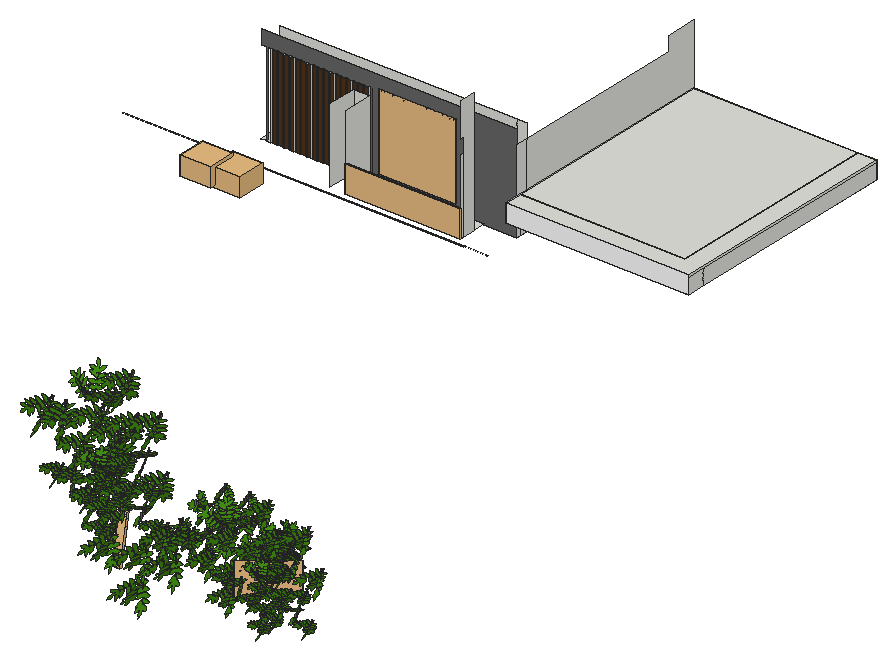
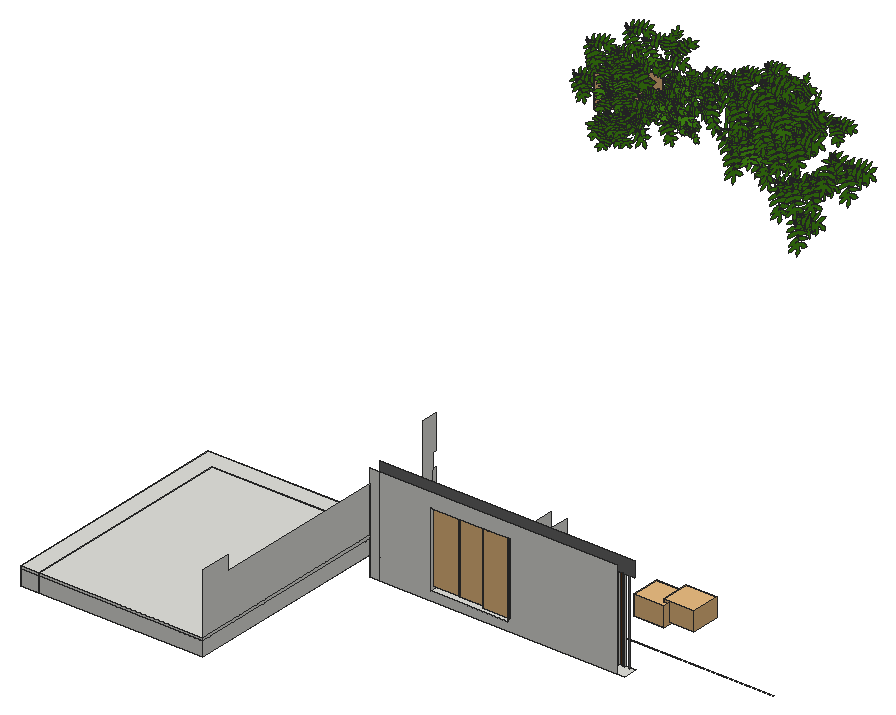
# SketchUp Ruby script. Lengths in inches.
U = 1.inch
M = Sketchup.active_model
def pt(a) = Geom::Point3d.new(a.map { |v| v * U })
def face(e, loops, mat)
  f = e.add_face(loops[0].map { |a| pt(a) })
  loops[1..].each { |l| e.add_face(l.map { |a| pt(a) }).erase! }
  f.material = f.back_material = mat if mat
  f
end
# faces: each face lists its corners as indices into pts; further lists are holes
def faces(e, pts, list, mat = nil) = list.each { |f| face(e, (f[0].is_a?(Array) ? f : [f]).map { |l| l.map { |i| pts[i] } }, mat) }
# xy, xz, yz: faces in a plane at the given z, y or x. An outline is a flat list of corners, or four numbers for a rectangle; further outlines are holes
def ring(l) = l.size == 4 ? [[l[0], l[1]], [l[2], l[1]], [l[2], l[3]], [l[0], l[3]]] : l.each_slice(2).to_a
def flat(e, list, mat, &to3) = list.each { |f| face(e, (f[0].is_a?(Array) ? f : [f]).map { |l| ring(l).map { |u, v| to3.(u, v) } }, mat) }
def xy(e, z, list, mat = nil) = flat(e, list, mat) { |x, y| [x, y, z] }
def xz(e, y, list, mat = nil) = flat(e, list, mat) { |x, z| [x, y, z] }
def yz(e, x, list, mat = nil) = flat(e, list, mat) { |y, z| [x, y, z] }
def lines(e, pts, list) = list.each { |a, b| e.add_line(pt(pts[a]), pt(pts[b])) }
# prism: a flat outline (further loops are holes) pulled along v
def prism(e, loops, v, mat = nil)
  f = face(e, loops, mat); d = Geom::Vector3d.new(v.map { |x| x * U })
  f.pushpull(f.normal.samedirection?(d) ? d.length : -d.length)
end
def box(e, o, s, mat = nil) = prism(e, [[o, [o[0] + s[0], o[1], o[2]], [o[0] + s[0], o[1] + s[1], o[2]], [o[0], o[1] + s[1], o[2]]]], [0, 0, s[2]], mat)
def at(x, y, z, deg = 0) = Geom::Transformation.translation(pt([x, y, z])) * Geom::Transformation.rotation(ORIGIN, Z_AXIS, deg.degrees)
def axes(o, x, y, z) = Geom::Transformation.new([*x, 0, *y, 0, *z, 0, *pt(o).to_a, 1])
def part(name) = M.definitions.add(name)
# library, detail: a bought-in or finely detailed component or shape, given as its bounding box
def library(name, o, s) = part(name).tap { |d| box(d.entities, o, s) }
def detail(e, o, s) = box(e.add_group.entities, o, s)
def put(e, d, t, mat = nil) = e.add_instance(d, t).tap { |i| i.material = mat if mat }
def group(e, t, mat = nil) = e.add_group.tap { |g| g.transformation = t; g.material = mat if mat }.entities
root = M.entities
M.materials.add("Material~3").color = [123, 113, 102]
M.materials.add("[0030_OldLace]").color = [86, 53, 24]
M.materials.add("[0128_White]").color = [255, 255, 255]
M.materials.add("[Slate Light Tile]").color = [104, 104, 104]
M.materials.add("[Wood Veneer 01]").color = [120, 70, 37]
M.materials.add("hojas").color = [70, 150, 19]
c1 = library("Ornamental+Grasses",[-8.33,-8.78,0],[17.11,15.88,10.63])
c2 = library("3DGeom~4_Defintion",[362.52,-15.59,12.6],[288.85,70.11,1000])
c3 = library("3 door",[0,0,0],[74.8,3.9375,43.31])
c4 = part("glass-railing")
detail(c4.entities,[0,0,0],[1.26,75.59,33.1875])
c5 = part("rama-acacia")
p = [[-13.53,0.69,-1.07],[-13.38,0.86,-0.98],[-13.61,0.85,-1.06],[-14.07,0.85,-1.21],[-15.17,0.86,-1.58],[-15.95,0.92,-1.83],
  [-16.01,1,-1.83],[-16.01,1.17,-1.78],[-16.07,1.93,-1.6],[-16.4,2.73,-1.5],[-16.65,3.06,-1.5],[-17.13,4.01,-1.41],
  [-17.78,4.7,-1.44],[-18.28,5.07,-1.51],[-18.57,5.18,-1.58],[-18.91,5.47,-1.62],[-19.07,5.48,-1.67],[-19.35,5.61,-1.73],
  [-19.51,5.64,-1.78],[-19.38,5.57,-1.75],[-19.33,5.5,-1.75],[-19.31,5.23,-1.82],[-19.38,5.08,-1.89],[-19.41,4.84,-1.96],
  [-19.36,4.59,-2.01],[-19.43,4.55,-2.04],[-19.36,4.15,-2.125],[-19.21,3.7,-2.19],[-18.875,3.1,-2.24],[-18.61,2.78,-2.24],
  [-17.83,2.19,-2.13],[-17.4375,1.85,-2.09],[-17.04,1.49,-2.05],[-16.61,1.24,-1.97],[-16.17,1.0625,-1.87],[-16.06,0.95,-1.86],
  [-16.06,0.91,-1.87],[-16.32,0.9,-1.96],[-16.7,0.88,-2.1],[-17.05,0.91,-2.21],[-17.61,1.15,-2.33],[-18.06,1.29,-2.45],
  [-18.88,1.53,-2.67],[-20.25,1.46,-3.15],[-20.59,1.49,-3.26],[-20.79,1.37,-3.36],[-21.08,1.2,-3.5],[-21.28,1.22,-3.5625],
  [-21.48,0.94,-3.71],[-21.79,0.5,-3.93],[-22.02,0.17,-4.1],[-22.11,0.05,-4.16],[-22.21,-0.02,-4.21],[-22.375,-0.05,-4.28],
  [-22.375,-0.07,-4.28],[-22.18,-0.09,-4.22],[-22.11,-0.07,-4.19],[-21.78,-0.1,-4.09],[-21.6,-0.18,-4.05],[-21.52,-0.27,-4.04],
  [-21.33,-0.33,-4],[-20.94,-0.54,-3.92],[-20.6875,-0.63,-3.86],[-20.54,-0.68,-3.82],[-20.42,-0.67,-3.78],[-20.09,-0.46,-3.61],
  [-19.8,-0.24,-3.45],[-19.21,-0.02,-3.19],[-18.48,0.08,-2.92],[-17.72,0.38,-2.58],[-17.4,0.5,-2.4375],[-16.93,0.75,-2.21],
  [-16.78,0.8,-2.15],[-16.1,0.83,-1.91],[-16.0625,0.81,-1.9],[-16.08,0.77,-1.91],[-16.27,0.72,-1.99],[-16.88,0.39,-2.29],
  [-17.1875,0.15,-2.46],[-17.27,0.02,-2.52],[-17.94,-0.52,-2.89],[-17.94,-0.59,-2.91],[-18.08,-0.68,-2.99],[-18.13,-0.86,-3.05],
  [-18.56,-1.55,-3.38],[-18.71,-2.11,-3.58],[-18.79,-2.61,-3.74],[-18.86,-2.84,-3.83],[-18.87,-3.07,-3.89],[-18.84,-3.22,-3.92],
  [-18.8,-3.26,-3.92],[-18.76,-3.47,-3.96],[-18.76,-3.6,-4],[-18.67,-3.8,-4.02],[-18.61,-3.92,-4.04],[-18.58,-4.11,-4.07],
  [-18.53,-4.18,-4.08],[-18.58,-4.35,-4.14],[-18.65,-4.43,-4.18],[-18.72,-4.51,-4.23],[-18.8125,-4.51,-4.26],[-18.8125,-4.53,-4.26],
  [-18.72,-4.54,-4.24],[-18.66,-4.49,-4.21],[-18.58,-4.43,-4.16],[-18.35,-4.23,-4.03],[-18.32,-4.17,-4],[-18.22,-4.125,-3.95],
  [-18.1,-4,-3.88],[-17.79,-3.72,-3.7],[-17.68,-3.51,-3.61],[-17.32,-3.13,-3.38],[-17.24,-2.94,-3.31],[-16.78,-2.12,-2.93],
  [-16.48,-1.78,-2.73],[-16.3,-1.28,-2.54],[-16.05,-0.75,-2.3125],[-15.89,-0.2,-2.11],[-15.89,0.39,-1.95],[-15.96,0.79,-1.87],
  [-15.91,0.82,-1.84],[-15.27,0.8,-1.63],[-14.18,0.76,-1.27],[-13.78,0.73,-1.15],[-13.78,0.67,-1.16],[-14.23,0.54,-1.35],
  [-14.65,0.33,-1.55],[-14.97,0.02,-1.74],[-15.25,-0.36,-1.9375],[-15.57,-0.72,-2.14],[-15.96,-1.64,-2.52],[-16.2,-2.51,-2.84],
  [-16.2,-3.12,-3],[-16.14,-3.41,-3.06],[-16.1,-3.75,-3.14],[-16.1,-4.09,-3.23],[-16.2,-4.25,-3.3],[-16.2,-4.28,-3.3125],
  [-16.08,-4.19,-3.24],[-15.98,-4.08,-3.18],[-15.96,-3.94,-3.14],[-15.96,-3.8125,-3.1],[-15.9,-3.72,-3.06],[-15.68,-3.55,-2.9375],
  [-15.51,-3.49,-2.86],[-15.3,-3.33,-2.75],[-15.23,-3.17,-2.68],[-15.01,-3.03,-2.57],[-14.875,-2.83,-2.47],[-14.6,-2.59,-2.3125],
  [-14.4,-2.27,-2.16],[-14.12,-1.6,-1.89],[-13.91,-1.1,-1.68],[-13.67,-0.83,-1.53],[-13.53,-0.45,-1.38],[-13.53,0.67,-1.08],
  [-12.41,6.01,0.65],[-12.44,6.14,0.68],[-12.41,6.29,0.73],[-12.43,6.29,0.73],[-12.44,6.26,0.72],[-12.47,6.15,0.68],
  [-12.49,6.07,0.66],[-12.57,5.75,0.55],[-12.67,5.36,0.43],[-12.79,4.875,0.28],[-12.83,4.52,0.18],[-12.83,3.99,0.04],
  [-12.73,3.11,-0.18],[-12.58,2.52,-0.3125],[-12.3,1.97,-0.41],[-11.88,1.51,-0.46],[-11.37,1.0625,-0.48],[-10.75,0.75,-0.45],
  [-10.75,0.68,-0.47],[-12.55,0.7,-0.79],[-13.21,0.79,-0.89],[-13.2,0.67,-0.92],[-12.56,0.62,-0.82],[-11.15,0.56,-0.58],
  [-10.79,0.54,-0.52],[-10.72,0.52,-0.51],[-10.72,0.5,-0.52],[-10.87,0.47,-0.55],[-11.14,0.41,-0.62],[-11.39,0.27,-0.7],
  [-11.625,-0.01,-0.82],[-11.8,-0.43,-0.96],[-11.83,-0.57,-1],[-12.02,-1.08,-1.17],[-12.1,-1.39,-1.27],[-12.17,-1.95,-1.4375],
  [-12.17,-2.77,-1.65],[-12.09,-3.59,-1.86],[-11.86,-4.26,-2],[-11.8125,-4.4,-2.03],[-11.84,-4.49,-2.05],[-11.91,-4.6,-2.1],
  [-11.97,-4.65,-2.12],[-11.98,-4.67,-2.13],[-11.92,-4.65,-2.11],[-11.84,-4.59,-2.08],[-11.77,-4.52,-2.05],[-11.74,-4.47,-2.03],
  [-11.37,-4.3125,-1.92],[-10.95,-4.0625,-1.78],[-10.82,-3.89,-1.71],[-10.64,-3.57,-1.59],[-10.41,-3.05,-1.41],[-10.27,-2.73,-1.3],
  [-10.07,-1.88,-1.03],[-10.15,-0.71,-0.73],[-10.31,-0.1,-0.6],[-10.5,0.4,-0.5],[-10.5,0.48,-0.48],[-10.44,0.53,-0.45],
  [-10.39,0.64,-0.42],[-10.52,0.73,-0.42],[-10.44,0.93,-0.35],[-10.44,1.2,-0.28],[-10.32,1.47,-0.18],[-10.48,2.6875,0.12],
  [-10.43,2.96,0.2],[-10.75,3.87,0.38],[-11.26,4.93,0.57],[-11.8,5.54,0.64],[-12.37,5.93,0.64],[-7.78,0.19,-0.06],
  [-7.78,0.25,-0.04],[-7.75,0.39,0],[-7.89,0.4,-0.02],[-7.96,0.46,-0.02],[-7.96,0.49,-0.01],[-7.76,0.62,0.06],
  [-7.53,0.99,0.2],[-7.31,1.78,0.45],[-7.31,2.74,0.71],[-7.63,3.6875,0.9],[-8.02,4.57,1.07],[-8.66,5.23,1.13],
  [-8.83,5.4,1.14],[-8.92,5.54,1.16],[-9.1,5.64,1.16],[-9.08,5.6,1.15],[-9.02,5.56,1.15],[-8.94,5.46,1.14],
  [-8.9,5.37,1.12],[-8.9375,5.25,1.08],[-9.14,4.92,0.96],[-9.31,4.5625,0.83],[-9.39,3.73,0.6],[-9.44,2.76,0.32],
  [-9.23,1.59,0.05],[-8.82,0.9,-0.06],[-8.36,0.59,-0.0625],[-8.14,0.51,-0.04],[-8.05,0.48,-0.03],[-8.05,0.46,-0.04],
  [-8.12,0.43,-0.06],[-10.1,0.49,-0.4],[-8.22,0.3125,-0.11],[-8.22,0.25,-0.125],[-8.53,0.13,-0.21],[-8.8,-0.16,-0.34],
  [-8.96,-0.61,-0.49],[-8.96,-0.87,-0.56],[-9.16,-1.42,-0.74],[-9.13,-1.77,-0.83],[-9.09,-1.83,-0.84],[-9.125,-1.92,-0.87],
  [-9.125,-2.13,-0.93],[-9.08,-2.23,-0.95],[-9.15,-2.39,-1],[-9.11,-2.67,-1.07],[-9.03,-2.86,-1.11],[-9.07,-3.03,-1.16],
  [-8.97,-3.23,-1.19],[-8.93,-3.44,-1.24],[-8.93,-3.71,-1.32],[-8.79,-4.05,-1.38],[-8.7,-4.25,-1.42],[-8.7,-4.39,-1.46],
  [-8.76,-4.53,-1.5],[-8.77,-4.65,-1.54],[-8.64,-4.55,-1.49],[-8.27,-4.22,-1.33],[-8.1875,-4.06,-1.27],[-8.07,-3.98,-1.23],
  [-7.98,-3.79,-1.17],[-7.79,-3.59,-1.08],[-7.64,-3.3,-0.97],[-7.64,-3.25,-0.96],[-7.59,-3.21,-0.9375],[-7.52,-2.93,-0.85],
  [-7.52,-2.85,-0.83],[-7.47,-2.81,-0.81],[-7.3,-2.09,-0.59],[-7.32,-2.01,-0.57],[-7.27,-1.95,-0.54],[-7.1875,-1.57,-0.42],
  [-7.17,-1.46,-0.39],[-7.17,-1.16,-0.3125],[-7.23,-0.61,-0.17],[-7.49,-0.15,-0.1],[-13.39,-0.07,-1.23],[-13.39,0.25,-1.14],
  [-13.49,0.5625,-1.09],[-13.8,1.01,-1.08],[-13.61,0.91,-1.04],[-13.38,0.92,-0.96],[-13.32,1.03,-0.91],[-13.32,1.35,-0.82],
  [-13.28,1.49,-0.77],[-13.28,1.99,-0.64],[-13.44,2.67,-0.51],[-13.72,3.31,-0.43],[-13.93,3.71,-0.4],[-14.1,4.39,-0.27],
  [-14.5625,5.06,-0.25],[-14.89,5.62,-0.21],[-15.33,6.1,-0.23],[-15.65,6.8,-0.15],[-15.79,6.89,-0.18],[-15.61,6.52,-0.22],
  [-15.51,6.32,-0.24],[-15.45,6.28,-0.23],[-15.52,6,-0.32],[-15.63,5.6875,-0.45],[-15.77,4.97,-0.68],[-15.7,4.25,-0.85],
  [-15.46,3,-1.11],[-15,2.03,-1.21],[-14.3,1.29,-1.17],[-4.5625,0.33,0.09],[-4.22,0.49,0.13],[-4,0.7,0.1875],
  [-3.86,0.99,0.26],[-3.77,1.41,0.38],[-3.7,1.73,0.46],[-3.77,1.99,0.53],[-3.85,2.17,0.58],[-3.88,2.57,0.6875],
  [-3.98,2.9,0.78],[-4.0625,2.97,0.8],[-4.1,3.14,0.84],[-4.1875,3.25,0.87],[-4.27,3.55,0.95],[-4.31,3.71,0.99],
  [-4.42,3.9,1.04],[-4.625,4.2,1.125],[-4.72,4.39,1.18],[-4.89,4.57,1.23],[-4.98,4.73,1.27],[-5,4.72,1.26],
  [-5.01,4.51,1.21],[-4.96,4.32,1.16],[-4.97,4.27,1.14],[-5.14,3.78,1.01],[-5.3,3.39,0.91],[-5.44,2.76,0.74],
  [-5.5,2.09,0.56],[-5.57,1.78,0.48],[-5.57,1.42,0.38],[-5.57,1.09,0.29],[-5.47,0.72,0.19],[-5.22,0.44,0.12],
  [-4.93,0.27,0.07],[-4.76,0.22,0.06],[-4.76,0.18,0.05],[-4.83,0.16,0.04],[-5.26,0,0],[-5.34,-0.04,-0.01],
  [-5.47,-0.22,-0.06],[-5.51,-0.6,-0.16],[-5.42,-1.09,-0.29],[-5.28,-1.49,-0.4],[-5.21,-1.87,-0.5],[-5.11,-2.15,-0.57],
  [-5.08,-2.34,-0.63],[-5.01,-2.47,-0.66],[-4.96,-2.69,-0.72],[-4.86,-2.9375,-0.79],[-4.84,-3.07,-0.82],[-4.77,-3.18,-0.85],
  [-4.74,-3.43,-0.92],[-4.7,-3.71,-0.99],[-4.62,-3.89,-1.04],[-4.58,-3.98,-1.07],[-4.58,-3.83,-1.03],[-4.51,-3.67,-0.98],
  [-4.3,-3.32,-0.89],[-4.16,-3.09,-0.83],[-4.16,-2.98,-0.8],[-4.11,-2.92,-0.78],[-4.02,-2.8,-0.75],[-3.95,-2.59,-0.69],
  [-3.95,-2.33,-0.625],[-3.86,-2.26,-0.6],[-3.86,-2.02,-0.54],[-3.86,-1.44,-0.39],[-3.94,-1.22,-0.33],[-3.94,-1.08,-0.29],
  [-4,-0.96,-0.26],[-4,-0.87,-0.23],[-4.0625,-0.8125,-0.22],[-4.16,-0.54,-0.14],[-4.39,-0.24,-0.06],[-4.61,-0.08,-0.02],
  [-4.77,-0.03,-0.01],[-4.77,-0.01,0],[-4.65,-0.01,0],[-4.61,0.19,0.05],[-4.66,0.23,0.0625],[-4.63,0.29,0.08],
  [-4.07,0.17,0.04],[0,-0.24,-0.06],[0,0,0],[-0.5,0.04,0.01],[-1.58,0.08,0.02],[-13.78,0.67,-1.08]]
faces(c5.entities,p,[[0,1,2,3,4,5,6,7,8,9,10,11,12,13,14,15,16,17,18,19,20,21,22,23,24,25,26,27,28,29,30,31,32,33,34,35,36,37,38,39,40,41,42,43,44,45,46,47,48,49,50,51,52,53,54,55,56,57,58,59,60,61,62,63,64,65,66,67,68,69,70,71,72,73,74,75,76,77,78,79,80,81,82,83,84,85,86,87,88,89,90,91,92,93,94,95,96,97,98,99,100,101,102,103,104,105,106,107,108,109,110,111,112,113,114,115,116,117,118,119,120,121,122,123,124,125,126,127,128,129,130,131,132,133,134,135,136,137,138,139,140,141,142,143,144,145,146,147,148,149,150,151,152,153,154,155],[156,157,158,159,160,161,162,163,164,165,166,167,168,169,170,171,172,173,174,175,176,177,178,179,180,181,182,183,184,185,186,187,188,189,190,191,192,193,194,195,196,197,198,199,200,201,202,203,204,205,206,207,208,209,210,211,212,213,214,215,216,217,218,219,220,221,222,223,224,225,226],[227,228,229,230,231,232,233,234,235,236,237,238,239,240,241,242,243,244,245,246,247,248,249,250,251,252,253,254,255,256,257,258,216,215,259,260,261,262,263,264,265,266,267,268,269,270,271,272,273,274,275,276,277,278,279,280,281,282,283,284,285,286,287,288,289,290,291,292,293,294,295,296,297,298,299,300,301,302,303],[154,304,305,306,155],[307,308,1,309,310,311,312,313,314,315,316,317,318,319,320,321,322,323,324,325,326,327,328,329,330,331,332],[333,334,335,336,337,338,339,340,341,342,343,344,345,346,347,348,349,350,351,352,353,354,355,356,357,358,359,360,361,362,363,364,365,366,367,368,369,370,371,372,373,374,375,376,377,378,379,380,381,382,383,384,385,386,387,388,389,390,391,392,393,394,395,396,397,398,399,400,401,402,403,404,405,406,407,408,409,410,411,412,413],[0,177,1],[308,2,1],
  [176,1,177],[414,411,410,415,416,417,418],[228,370,229],[369,229,370]],"hojas")
lines(c5.entities,p,[[155,419]])
c6 = part("Group\#150")
put(c6.entities,c5,axes([10.13,10.27,0],[0.45315,0.21131,0],[-0.21131,0.45315,0],[0,0,0.5]))
put(c6.entities,c5,axes([10.13,10.27,0],[0.11638,0.47539,0.10227],[-0.48087,0.12813,-0.0484],[-0.07223,-0.08709,0.48703]))
put(c6.entities,c5,axes([9.58,10.26,-0.7],[0.1449,0.38901,-0.2787],[-0.10883,0.31035,0.37662],[0.46601,-0.04848,0.17461]))
c7 = part("Group\#151")
put(c7.entities,c6,axes([24.99,4.24,9.59],[0.78856,0.61496,0],[0.01473,-0.01889,0.99971],[0.61478,-0.78833,-0.02396]))
put(c7.entities,c6,axes([39.5,6.625,12.55],[0.6544,0.49291,0.57341],[-0.44023,-0.3682,0.81892],[0.61478,-0.78833,-0.02396]))
put(c7.entities,c6,axes([32.34,3.7,6.88],[0.78856,0.61496,0],[0.01473,-0.01889,0.99971],[0.61478,-0.78833,-0.02396]))
put(c7.entities,c6,axes([43.14,6.65,17.54],[0.78856,0.61496,0],[0.35273,-0.4523,0.81915],[0.50374,-0.64595,-0.57358]))
put(c7.entities,c6,axes([12.2,6.2,16.68],[0.7209,0.54936,0.4225],[-0.31991,-0.27701,0.90605],[0.61478,-0.78833,-0.02396]))
put(c7.entities,c6,axes([49.9375,3.79,26.09],[0.78856,0.61496,0],[0.01473,-0.01889,0.99971],[0.61478,-0.78833,-0.02396]))
put(c7.entities,c6,axes([36.11,4.9375,33.94],[0.78856,0.61496,0],[0.01473,-0.01889,0.99971],[0.61478,-0.78833,-0.02396]))
put(c7.entities,c6,axes([39.61,3.79,23.47],[0.78856,0.61496,0],[0.01473,-0.01889,0.99971],[0.61478,-0.78833,-0.02396]))
put(c7.entities,c6,axes([25.59,6.5625,46.47],[-0.40704,-0.29112,-0.86578],[0.67555,0.54201,-0.49986],[0.61478,-0.78833,-0.02396]))
put(c7.entities,c6,axes([54.97,1.98,11.65],[0.78856,0.61496,0],[0.01473,-0.01889,0.99971],[0.61478,-0.78833,-0.02396]))
put(c7.entities,c6,axes([32.97,3.79,19.14],[0.78856,0.61496,0],[0.01473,-0.01889,0.99971],[0.61478,-0.78833,-0.02396]))
put(c7.entities,c6,axes([24.24,3.79,21.99],[0.78856,0.61496,0],[0.01473,-0.01889,0.99971],[0.61478,-0.78833,-0.02396]))
put(c7.entities,c6,axes([16.86,4.24,12.3],[0.78856,0.61496,0],[0.01473,-0.01889,0.99971],[0.61478,-0.78833,-0.02396]))
put(c7.entities,c6,axes([1.23,3.9375,19.07],[0.78856,0.61496,0],[0.01473,-0.01889,0.99971],[0.61478,-0.78833,-0.02396]))
put(c7.entities,c6,axes([29.05,5.25,29.11],[0.78856,0.61496,0],[0.21033,-0.2697,0.93969],[0.57787,-0.741,-0.34202]))
put(c7.entities,c6,axes([24.16,3.79,-0.1],[0.78856,0.61496,0],[0.01473,-0.01889,0.99971],[0.61478,-0.78833,-0.02396]))
c8 = library("Group\#154",[0,0,0],[9.94,2.45,66.78])
c9 = library("Group\#152",[0,0,0],[130.24,0.88,39.6])
xy(root,162.75,[[2170.98,845.35,2587.8,846.1],[2396.11,888.83,2396.11,890.39,2394.52,890.39,2394.52,888.95,2389.11,888.95,2389.11,890.39,2387.52,890.39,2387.52,888.95,2382.11,888.95,2382.11,890.39,2380.52,890.39,2380.52,888.95,2375.11,888.95,2375.11,890.39,2373.52,890.39,2373.52,888.95,2368.11,888.95,2368.11,890.39,2366.52,890.39,2366.52,888.95,2361.11,888.95,2361.11,890.39,2359.52,890.39,2359.52,888.95,2354.11,888.95,2354.11,890.39,2352.52,890.39,2352.52,888.95,2347.11,888.95,2347.11,890.39,2345.52,890.39,2345.52,888.95,2340.11,888.95,2340.11,890.39,2338.52,890.39,2338.52,888.95,2333.11,888.95,2333.11,890.39,2331.52,890.39,2331.52,888.95,2326.11,888.95,2326.11,890.39,2324.52,890.39,2324.52,888.95,2319.11,888.95,2319.11,890.39,2317.52,890.39,2317.52,888.95,2312.11,888.95,2312.11,890.39,2310.46,890.39,2310.46,888.95,2305.05,888.95,2305.05,905.7,2617.01,905.7,2617.01,890.39,2436.52,890.39,2436.52,888.83,2431.11,888.83,2431.11,890.39,2429.52,890.39,2429.52,888.83,2424.11,888.83,2424.11,890.39,2422.52,890.39,2422.52,888.83,2417.11,888.83,2417.11,890.39,2415.52,890.39,2415.52,888.83,2410.11,888.83,2410.11,890.39,2408.52,890.39,2408.52,888.83,2403.11,888.83,2403.11,890.39,2401.52,890.39,2401.52,888.83]])
xy(root,163,[[2587.8,845.35,2617.01,846.1]])
xy(root,173.4375,[[2447.38,840.97,2587.8,877.14],[2447.58,890.39,2542.64,905.7]])
xy(root,186.75,[[2803.93,893.65,2810.07,895.71],[2812.24,893.65,2818.39,895.71],[2621.05,894.34,2627.2,895.71],[2629.36,894.34,2635.51,895.71],[2637.68,894.34,2643.82,895.71],
  [2645.99,894.34,2652.14,895.71],[2654.3,894.34,2660.45,895.71],[2662.61,894.34,2668.76,895.71],[2670.93,894.34,2677.07,895.71],[2679.24,894.34,2685.39,895.71],
  [2687.55,894.34,2693.7,895.71],[2695.86,894.34,2702.01,895.71],[2704.18,894.34,2710.32,895.71],[2712.49,894.34,2718.64,895.71],[2720.8,894.34,2726.95,895.71],
  [2729.11,894.34,2735.26,895.71],[2737.43,894.34,2743.57,895.71],[2745.74,894.34,2751.89,895.71],[2754.05,894.34,2760.2,895.71],[2762.36,894.34,2768.51,895.71],
  [2770.68,894.34,2776.82,895.71],[2778.99,894.34,2785.14,895.71],[2787.3,894.34,2793.45,895.71],[2795.61,894.34,2801.76,895.71],[[2617.01,895.71,2818.39,1160.85],[2625.48,904.18,2807.17,1152.375]]])
xy(root,186.75,[[2617.01,873.28,2617.01,895.71,2621.05,895.71,2621.05,894.34,2627.2,894.34,2627.2,895.71,2629.36,895.71,2629.36,894.34,2635.51,894.34,2635.51,895.71,2637.68,895.71,2637.68,894.34,2643.82,894.34,2643.82,895.71,2645.99,895.71,2645.99,894.34,2652.14,894.34,2652.14,895.71,2654.3,895.71,2654.3,894.34,2660.45,894.34,2660.45,895.71,2662.61,895.71,2662.61,894.34,2668.76,894.34,2668.76,895.71,2670.93,895.71,2670.93,894.34,2677.07,894.34,2677.07,895.71,2679.24,895.71,2679.24,894.34,2685.39,894.34,2685.39,895.71,2687.55,895.71,2687.55,894.34,2693.7,894.34,2693.7,895.71,2695.86,895.71,2695.86,894.34,2702.01,894.34,2702.01,895.71,2704.18,895.71,2704.18,894.34,2710.32,894.34,2710.32,895.71,2712.49,895.71,2712.49,894.34,2718.64,894.34,2718.64,895.71,2720.8,895.71,2720.8,894.34,2726.95,894.34,2726.95,895.71,2729.11,895.71,2729.11,894.34,2735.26,894.34,2735.26,895.71,2737.43,895.71,2737.43,894.34,2743.57,894.34,2743.57,895.71,2745.74,895.71,2745.74,894.34,2751.89,894.34,2751.89,895.71,2754.05,895.71,2754.05,894.34,2760.2,894.34,2760.2,895.71,2762.36,895.71,2762.36,894.34,2768.51,894.34,2768.51,895.71,2770.68,895.71,2770.68,894.34,2776.82,894.34,2776.82,895.71,2778.99,895.71,2778.99,894.34,2785.14,894.34,2785.14,895.71,2787.3,895.71,2787.3,894.34,2793.45,894.34,2793.45,895.71,2795.61,895.71,2795.61,894.34,2801.76,894.34,2801.76,895.71,2803.93,895.71,2803.93,893.65,2810.07,893.65,2810.07,895.71,2812.24,895.71,2812.24,893.65,2818.39,893.65,2818.39,895.71,2840.8125,895.71,2840.8125,873.28],[2818.39,895.71,2840.8125,1160.85]],"[Wood Veneer 01]")
xy(root,204.8125,[[[2617.01,895.71,2818.39,1160.85],[2625.48,904.18,2807.17,1152.375]],[2818.39,895.71,2840.8125,1160.85]])
xy(root,208.375,[[2617.01,873.28,2840.8125,873.28,2840.8125,1160.85,2818.39,1160.85,2818.39,895.71,2617.01,895.71],[2617.01,895.71,2818.39,1160.85]])
xz(root,873.28,[[2617.01,186.75,2840.8125,208.375]],"[0128_White]")
xz(root,877.14,[[2427.73,173.4375,2447.38,264.75]])
xz(root,888.83,[[2396.11,162.75,2401.52,264.75],[2403.11,162.75,2408.52,264.75],[2410.11,162.75,2415.52,264.75],[2417.11,162.75,2422.52,264.75],[2424.11,162.75,2429.52,264.75],
  [2431.11,162.75,2436.52,264.75]],"[0030_OldLace]")
xz(root,888.95,[[2319.11,162.75,2324.52,264.75],[2326.11,162.75,2331.52,264.75],[2333.11,162.75,2338.52,264.75],[2340.11,162.75,2345.52,264.75],[2347.11,162.75,2352.52,264.75],
  [2354.11,162.75,2359.52,264.75],[2361.11,162.75,2366.52,264.75],[2368.11,162.75,2373.52,264.75],[2375.11,162.75,2380.52,264.75],[2382.11,162.75,2387.52,264.75],
  [2389.11,162.75,2394.52,264.75]],"[0030_OldLace]")
xz(root,890.39,[[[2310.46,162.75,2312.11,162.75,2312.11,264.75,2317.52,264.75,2317.52,162.75,2319.11,162.75,2319.11,264.75,2324.52,264.75,2324.52,162.75,2326.11,162.75,2326.11,264.75,2331.52,264.75,2331.52,162.75,2333.11,162.75,2333.11,264.75,2338.52,264.75,2338.52,162.75,2340.11,162.75,2340.11,264.75,2345.52,264.75,2345.52,162.75,2347.11,162.75,2347.11,264.75,2352.52,264.75,2352.52,162.75,2354.11,162.75,2354.11,264.75,2359.52,264.75,2359.52,162.75,2361.11,162.75,2361.11,264.75,2366.52,264.75,2366.52,162.75,2368.11,162.75,2368.11,264.75,2373.52,264.75,2373.52,162.75,2375.11,162.75,2375.11,264.75,2380.52,264.75,2380.52,162.75,2382.11,162.75,2382.11,264.75,2387.52,264.75,2387.52,162.75,2389.11,162.75,2389.11,264.75,2394.52,264.75,2394.52,162.75,2396.11,162.75,2396.11,264.75,2401.52,264.75,2401.52,162.75,2403.11,162.75,2403.11,264.75,2408.52,264.75,2408.52,162.75,2410.11,162.75,2410.11,264.75,2415.52,264.75,2415.52,162.75,2417.11,162.75,2417.11,264.75,2422.52,264.75,2422.52,162.75,2424.11,162.75,2424.11,264.75,2429.52,264.75,2429.52,162.75,2431.11,162.75,2431.11,264.75,2436.52,264.75,2436.52,162.75,2617.01,162.75,2617.01,282.75,2305.05,282.75,2305.05,264.75,2310.46,264.75],[2447.58,173.4375,2542.64,264.75]]],"[Slate Light Tile]")
xz(root,895.71,[[2617.01,186.75,2818.39,204.8125],[2818.39,186.75,2840.8125,204.8125],[2617.01,204.8125,2818.39,208.375]])
xz(root,904.18,[[2625.48,186.75,2807.17,204.8125]])
xz(root,905.7,[[[2314.43,162.75,2604.75,282.75],[2447.58,173.4375,2542.64,264.75]],[2604.75,162.75,2617.01,282.75]])
xz(root,1152.375,[[2625.48,186.75,2807.17,204.8125]])
xz(root,1160.85,[[2617.01,186.75,2818.39,204.8125],[2818.39,186.75,2840.8125,204.8125],[2617.01,204.8125,2818.39,208.375],[2818.39,204.8125,2840.8125,208.375]])
yz(root,2317.52,[[888.95,162.75,890.39,264.75]])
yz(root,2319.11,[[888.95,162.75,890.39,264.75]])
yz(root,2324.52,[[888.95,162.75,890.39,264.75]])
yz(root,2326.11,[[888.95,162.75,890.39,264.75]])
yz(root,2331.52,[[888.95,162.75,890.39,264.75]])
yz(root,2333.11,[[888.95,162.75,890.39,264.75]])
yz(root,2338.52,[[888.95,162.75,890.39,264.75]])
yz(root,2340.11,[[888.95,162.75,890.39,264.75]])
yz(root,2345.52,[[888.95,162.75,890.39,264.75]])
yz(root,2347.11,[[888.95,162.75,890.39,264.75]])
yz(root,2352.52,[[888.95,162.75,890.39,264.75]])
yz(root,2354.11,[[888.95,162.75,890.39,264.75]])
yz(root,2359.52,[[888.95,162.75,890.39,264.75]])
yz(root,2361.11,[[888.95,162.75,890.39,264.75]])
yz(root,2366.52,[[888.95,162.75,890.39,264.75]])
yz(root,2368.11,[[888.95,162.75,890.39,264.75]])
yz(root,2373.52,[[888.95,162.75,890.39,264.75]])
yz(root,2375.11,[[888.95,162.75,890.39,264.75]])
yz(root,2380.52,[[888.95,162.75,890.39,264.75]])
yz(root,2382.11,[[888.95,162.75,890.39,264.75]])
yz(root,2387.52,[[888.95,162.75,890.39,264.75]])
yz(root,2389.11,[[888.95,162.75,890.39,264.75]])
yz(root,2394.52,[[888.95,162.75,890.39,264.75]])
yz(root,2396.11,[[888.83,162.75,890.39,264.75]])
yz(root,2401.52,[[888.83,162.75,890.39,264.75]])
yz(root,2403.11,[[888.83,162.75,890.39,264.75]])
yz(root,2408.52,[[888.83,162.75,890.39,264.75]])
yz(root,2410.11,[[888.83,162.75,890.39,264.75]],"[0030_OldLace]")
yz(root,2415.52,[[888.83,162.75,890.39,264.75]])
yz(root,2417.11,[[888.83,162.75,890.39,264.75]],"[0030_OldLace]")
yz(root,2422.52,[[888.83,162.75,890.39,264.75]])
yz(root,2424.11,[[888.83,162.75,890.39,264.75]],"[0030_OldLace]")
yz(root,2427.73,[[840.97,173.4375,877.14,264.75]])
yz(root,2429.52,[[888.83,162.75,890.39,264.75]])
yz(root,2431.11,[[888.83,162.75,890.39,264.75]],"[0030_OldLace]")
yz(root,2436.52,[[888.83,162.75,890.39,264.75]])
yz(root,2447.38,[[840.97,173.4375,877.14,264.75]])
yz(root,2447.58,[[890.39,173.4375,905.7,264.75]])
yz(root,2542.64,[[890.39,173.4375,905.7,264.75]])
yz(root,2587.8,[[845.35,162.75,846.1,163],[840.97,173.4375,846.1,264.75],[846.1,173.4375,846.1,264.75,845.35,264.75,845.35,282.75,840.97,282.75,840.97,324.5625,861.24,324.5625,861.24,173.4375]])
yz(root,2617.01,[[890.39,162.75,895.71,186.75],[895.71,162.75,905.7,186.75],[873.28,186.75,890.39,204.8125],[890.39,186.75,895.71,204.8125],[895.71,186.75,905.7,204.8125],
  [905.7,186.75,1160.85,204.8125],[873.28,204.8125,890.39,208.375],[890.39,204.8125,895.71,208.375],[895.71,204.8125,905.7,208.375],[905.7,204.8125,1160.85,208.375],
  [890.39,208.375,905.7,264.75],[905.7,208.375,1160.85,208.375,1160.85,282.75,1122.97,282.75,1122.97,264.75,905.7,264.75]])
yz(root,2625.48,[[904.18,186.75,905.7,204.8125],[905.7,186.75,1152.375,204.8125]])
yz(root,2807.17,[[904.18,186.75,1152.375,204.8125]])
yz(root,2818.39,[[895.71,186.75,1160.85,204.8125],[895.71,204.8125,1160.85,208.375]])
yz(root,2840.8125,[[873.28,186.75,895.71,204.8125],[895.71,186.75,1160.85,204.8125],[873.28,204.8125,1160.85,208.375]])
p = [[2439.68,890.39,264.75],[2439.68,890.39,162.75]]
lines(root,p,[[0,1]])
put(root,c1,axes([2317.21,791.57,170.63],[2.19,0,0],[0,2.19,0],[0,0,2.19]))
put(root,c1,axes([2348.36,798.1875,167.75],[2.19,0,0],[0,2.19,0],[0,0,2.19]))
put(root,c2,axes([2405.72,905.3125,176.31],[0.11056,0,0],[0,-0.05859,0],[0,0,0.08734]),"Material~3")
put(root,c2,axes([2437.32,901.24,176.31],[0.11056,0,0],[0,-0.05859,0],[0,0,0.08734]),"Material~3")
put(root,c3,axes([2447.58,890.39,173.4375],[1.27084,0,0],[0,1.38,0],[0,0,2.15904]))
put(root,c4,axes([2447.32,841,173.4375],[0,-1,0],[1.86,0,0],[0,0,1]))
put(root,c2,axes([2470.63,901.24,176.31],[0.11056,0,0],[0,-0.05859,0],[0,0,0.08734]),"Material~3")
put(root,c7,axes([2589.79,143.6,183.16],[2.73544,0,0],[0,3.9644,0],[0,0,3.9644]))
put(root,c7,axes([2669.375,81.6875,217.875],[2.32,0,0],[0,2.32,0],[0,0,2.32]))
put(root,c8,axes([2759.76,91.79,203.72],[0.99668,0.06114,0.0538],[-0.04369,0.95891,-0.28031],[-0.06873,0.27703,0.9584]))
put(root,c6,axes([2766.65,38.93,216.24],[0.80931,3.79087,0],[0.09082,-0.01939,3.87519],[3.78978,-0.80908,-0.09287]))
put(root,c6,axes([2789.45,55.78,168.17],[0.80931,3.79087,0],[0.09082,-0.01939,3.87519],[3.78978,-0.80908,-0.09287]))
put(root,c6,axes([2790.8125,59.21,205.76],[0.80931,3.79087,0],[0.09082,-0.01939,3.87519],[3.78978,-0.80908,-0.09287]))
put(root,c6,axes([2813.96,75.89,195.25],[0.80931,3.79087,0],[0.09082,-0.01939,3.87519],[3.78978,-0.80908,-0.09287]))
put(root,c6,axes([2827.95,102.4375,217.24],[0.71504,3.09418,2.22272],[-0.38981,-2.19024,3.17437],[3.78978,-0.80908,-0.09287]))
put(root,c7,axes([2834.99,74.22,219.39],[0.75649,1.62229,0],[-1.62229,0.75649,0],[0,0,1.79]))
put(root,c6,axes([2838.6875,111.58,236.57],[0.80931,3.79087,0],[2.17436,-0.4642,3.17528],[3.1053,-0.66295,-2.22335]))
put(root,c6,axes([2885.45,127.2,213.73],[0.80931,3.79087,0],[0.09082,-0.01939,3.87519],[3.78978,-0.80908,-0.09287]))
put(root,c7,axes([2825.17,46.91,192.17],[2.57391,1.20024,0],[-1.20024,2.57391,0],[0,0,2.84]))
put(root,c7,axes([2867.25,192.19,197.57],[0.905,-1.56751,0],[2.89989,1.67425,0],[0,0,1.81]))
put(root,c9,axes([2906.23,96.49,218.68],[0.39163,0.31085,0],[-0.12434,0.15665,0],[0,0,1]))
put(root,c7,axes([2882.05,82.51,184.23],[1.9,0,0],[0,1.9,0],[0,0,1.9]))
